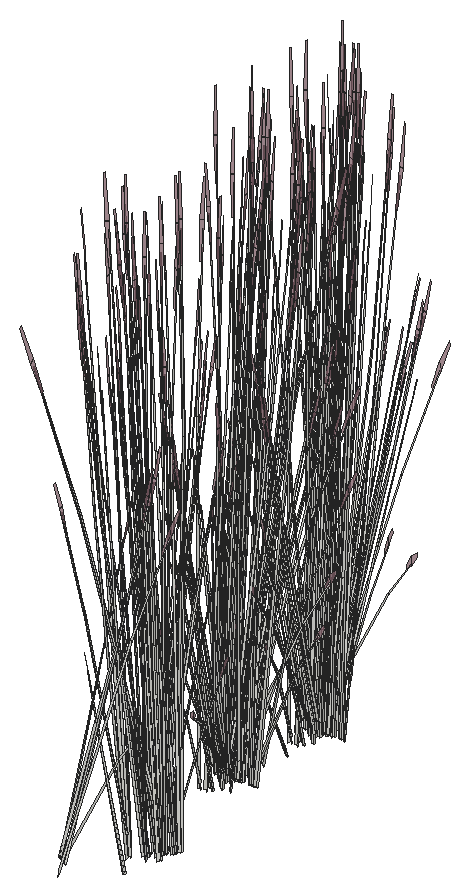
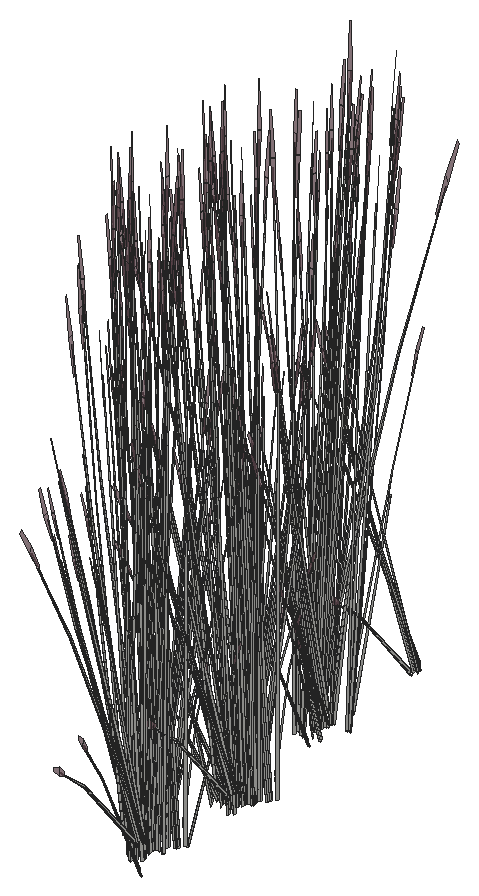
# SketchUp Ruby script. Lengths in inches.
U = 1.inch
M = Sketchup.active_model
def pt(a) = Geom::Point3d.new(a.map { |v| v * U })
def face(e, loops, mat)
  f = e.add_face(loops[0].map { |a| pt(a) })
  loops[1..].each { |l| e.add_face(l.map { |a| pt(a) }).erase! }
  f.material = f.back_material = mat if mat
  f
end
# faces: each face lists its corners as indices into pts; further lists are holes
def faces(e, pts, list, mat = nil) = list.each { |f| face(e, (f[0].is_a?(Array) ? f : [f]).map { |l| l.map { |i| pts[i] } }, mat) }
# xy, xz, yz: faces in a plane at the given z, y or x. An outline is a flat list of corners, or four numbers for a rectangle; further outlines are holes
def ring(l) = l.size == 4 ? [[l[0], l[1]], [l[2], l[1]], [l[2], l[3]], [l[0], l[3]]] : l.each_slice(2).to_a
def flat(e, list, mat, &to3) = list.each { |f| face(e, (f[0].is_a?(Array) ? f : [f]).map { |l| ring(l).map { |u, v| to3.(u, v) } }, mat) }
def xy(e, z, list, mat = nil) = flat(e, list, mat) { |x, y| [x, y, z] }
def xz(e, y, list, mat = nil) = flat(e, list, mat) { |x, z| [x, y, z] }
def yz(e, x, list, mat = nil) = flat(e, list, mat) { |y, z| [x, y, z] }
def lines(e, pts, list) = list.each { |a, b| e.add_line(pt(pts[a]), pt(pts[b])) }
# prism: a flat outline (further loops are holes) pulled along v
def prism(e, loops, v, mat = nil)
  f = face(e, loops, mat); d = Geom::Vector3d.new(v.map { |x| x * U })
  f.pushpull(f.normal.samedirection?(d) ? d.length : -d.length)
end
def box(e, o, s, mat = nil) = prism(e, [[o, [o[0] + s[0], o[1], o[2]], [o[0] + s[0], o[1] + s[1], o[2]], [o[0], o[1] + s[1], o[2]]]], [0, 0, s[2]], mat)
def at(x, y, z, deg = 0) = Geom::Transformation.translation(pt([x, y, z])) * Geom::Transformation.rotation(ORIGIN, Z_AXIS, deg.degrees)
def axes(o, x, y, z) = Geom::Transformation.new([*x, 0, *y, 0, *z, 0, *pt(o).to_a, 1])
def part(name) = M.definitions.add(name)
# library, detail: a bought-in or finely detailed component or shape, given as its bounding box
def library(name, o, s) = part(name).tap { |d| box(d.entities, o, s) }
def detail(e, o, s) = box(e.add_group.entities, o, s)
def put(e, d, t, mat = nil) = e.add_instance(d, t).tap { |i| i.material = mat if mat }
def group(e, t, mat = nil) = e.add_group.tap { |g| g.transformation = t; g.material = mat if mat }.entities
root = M.entities
M.materials.add("LightPink_Translucent").color = [144, 107, 117]
M.materials["LightPink_Translucent"].alpha = 0.75
c1 = part("blade")
p = [[2.15,0.21,22],[0,0.17,0],[0.09,0.45,0],[2.18,0.31,22],[2.29,0.31,22],[0.38,0.45,0],
  [2.48,0.24,33],[2.49,0.24,33],[2.48,0.22,33]]
faces(c1.entities,p,[[0,1,2,3],[4,5,2,3],[6,3,4,7],[8,0,3,6]])
c2 = part("seeds")
p = [[0.3,-0.1,1.38],[-0.01,-0.03,1.59],[-0.01,-0.03,0.03],[0.14,-0.07,-0.07],[0.29,-0.03,3],[0.15,0.01,3.11]]
faces(c2.entities,p,[[0,1,2,3],[1,0,4,5]],"LightPink_Translucent")
c3 = part("blade with seeds")
put(c3.entities,c1,at(0,0,0))
put(c3.entities,c2,axes([2.4,0.25,30.99],[1.5799,-0.05474,1.17369],[-0.12525,1.92788,0.29478],[-0.07173,-0.02425,1.56792]))
put(root,c3,axes([405.5625,393.34,-10.02],[-0.35341,0.31182,-0.03625],[-0.32382,-0.34152,-0.16435],[-0.0228,-0.09677,0.54209]))
put(root,c3,axes([403.33,388.5,-7.64],[0.50273,0.13626,-0.47583],[-0.17232,0.46717,-0.36857],[0.0461,0.18809,0.91046]))
put(root,c3,axes([403.61,387.54,-8.39],[-0.1169,-0.17452,1.59586],[0.54019,-0.14692,0.12904],[0.12209,0.27397,0.68222]))
put(root,c3,axes([406.02,397.03,-8.9],[0.44194,0.21918,1.40854],[-0.43295,0.47219,0.557],[-0.19393,-0.27986,1.18082]))
put(root,c3,axes([403.1,388.79,-7.78],[-0.15418,0.41799,-0.32977],[-0.44981,-0.12192,0.42575],[0.04124,0.16829,0.81462]))
put(root,c3,axes([405.09,394.07,-7.3],[0.07899,0.43781,0.32977],[-0.45153,0.11561,-0.42575],[-0.12128,-0.12546,0.81462]))
put(root,c3,axes([403.71,395.52,-10.12],[0,-0.54355,-0.46235],[0.57217,0,0],[0,-0.1238,1.46668]))
put(root,c3,axes([403.14,388.41,-7.36],[0.24409,0.44196,-0.66157],[-0.50245,0.2463,0.07984],[0.05708,0.21354,0.93586]))
put(root,c3,axes([405.26,395.74,-9.94],[0.24813,-0.48978,-0.41661],[0.51557,0.23571,0.2005],[0,-0.1129,1.33761]))
put(root,c3,axes([403.95,395.53,-10.11],[0.35699,-0.33913,-0.28847],[0.35699,0.33913,0.28847],[0,-0.10923,1.29413]))
put(root,c3,axes([402.78,389.53,-7.61],[0.06483,0.08753,1.62908],[0.52315,0.03439,-0.25764],[0.05261,0.19303,0.13065]))
put(root,c3,axes([405.2,396.15,-9.52],[-0.57594,-0.25935,-0.27094],[0.27732,-0.5474,-0.46562],[-0.0181,-0.1344,1.4872]))
put(root,c3,axes([404.06,395.77,-9.83],[-0.47569,0.45698,0.2864],[-0.47598,-0.45217,-0.33981],[-0.01661,-0.12977,1.53541]))
put(root,c3,axes([405.35,396.72,-9.73],[0.13555,-0.64407,-0.21817],[0.64269,0.11227,0.47743],[-0.1123,-0.08895,1.45677]))
put(root,c3,axes([403.95,396.02,-9.69],[0,0.54355,0.46235],[-0.57217,0,0],[0,-0.1238,1.46668]))
put(root,c3,axes([405.3,396.46,-9.94],[-0.30722,-0.45622,-0.41661],[0.46535,-0.32126,0.2005],[-0.09942,-0.05645,1.33761]))
put(root,c3,axes([405.37,395.82,-9.8],[0.22235,0.6078,0.42607],[-0.63531,0.21135,0.16719],[0.00776,-0.11168,1.47927]))
put(root,c3,axes([405.25,396.3,-9.47],[-0.24813,0.48978,0.41661],[-0.51557,-0.23571,-0.2005],[0,-0.1129,1.33761]))
put(root,c3,axes([406.33,396.36,-9.86],[-0.47569,-0.46784,-0.05709],[0.47598,-0.46812,0],[-0.01661,-0.01634,1.63492]))
put(root,c3,axes([405.42,396.41,-9.8],[0.64638,0.11452,0.42607],[-0.13155,0.64678,0.16719],[-0.09446,-0.06245,1.47927]))
put(root,c3,axes([405.07,397.45,-9.7],[0.54955,-0.14427,0.16428],[0.1357,0.53689,0.32672],[-0.04901,-0.07823,1.49371]))
put(root,c3,axes([405.9,397.32,-9.95],[-0.16686,-0.46861,0],[0.47648,-0.16411,0],[0,0,1.4375]))
put(root,c3,axes([405.58,396.875,-9.5625],[-0.09866,0.48509,0.13483],[-0.48202,-0.0842,-0.38503],[-0.08772,-0.04981,1.18024]))
put(root,c3,axes([406.71,397.48,-9.7],[0.14774,-0.54019,0.16428],[0.54062,0.15287,0.32672],[-0.09339,0.00263,1.49371]))
put(root,c3,axes([405.78,397.53,-9.95],[-0.51557,-0.24403,0],[0.24813,-0.50705,0],[0,0,1.51513]))
put(root,c3,axes([406.21,396.88,-9.7],[-0.49938,-0.43748,-0.23459],[0.42021,-0.49126,0.51337],[-0.13447,0.05118,1.56642]))
put(root,c3,axes([404.9,397.72,-9.69],[0.47863,0.27177,0.46235],[-0.28609,0.48733,0],[-0.10901,-0.0619,1.46668]))
put(root,c3,axes([406.45,396.52,-9.47],[0.55535,-0.03355,0.41661],[0.05022,0.55698,-0.2005],[-0.09942,0.05645,1.33761]))
put(root,c3,axes([405.96,396.79,-9.94],[-0.55535,0.03355,-0.41661],[-0.05022,-0.55698,0.2005],[-0.09942,0.05645,1.33761]))
put(root,c3,axes([406.57,398.08,-9.96],[-0.31576,-0.54657,-0.04789],[0.53494,-0.30375,0.48057],[-0.13182,0.05204,1.52373]))
put(root,c3,axes([406.46,396.76,-9.5625],[0.37783,0.32657,0.13483],[-0.31516,0.36844,-0.38503],[-0.08772,0.04981,1.18024]))
put(root,c3,axes([406.86,397.76,-9.69],[0.47863,-0.27177,0.46235],[0.28609,0.48733,0],[-0.10901,0.0619,1.46668]))
put(root,c3,axes([406.43,398.01,-10.11],[-0.47712,-0.13449,-0.28847],[0.12013,-0.47362,0.28847],[-0.09619,0.05462,1.29413]))
put(root,c3,axes([406.35,396.64,-9.52],[0.05959,0.62022,-0.27094],[-0.62068,0.0375,-0.46562],[-0.1093,0.08261,1.4872]))
put(root,c3,axes([406.57,396.4,-9.94],[-0.24813,0.48978,-0.41661],[-0.51557,-0.23571,0.2005],[0,0.1129,1.33761]))
put(root,c3,axes([405.97,397.11,-10.08],[-0.34446,0.40855,-0.58063],[-0.42791,-0.37046,-0.15239],[-0.13803,0.10191,1.28164]))
put(root,c3,axes([406.59,397.8,-9.83],[0.64025,0.17667,0.2864],[-0.16018,0.63149,-0.33981],[-0.10597,0.07904,1.53541]))
put(root,c3,axes([406.54,398.23,-10.12],[-0.47863,0.27177,-0.46235],[-0.28609,-0.48733,0],[-0.10901,0.0619,1.46668]))
put(root,c3,axes([404.38,397.5625,-7.3],[0.34603,-0.28618,0.32977],[0.32756,0.32677,-0.42575],[-0.04984,0.16603,0.81462]))
put(root,c3,axes([406.98,398.14,-9.79],[0.31974,0.54466,0],[-0.53494,0.30375,-0.48057],[-0.12184,0.06918,1.52448]))
put(root,c3,axes([406.7,395.99,-9.35],[-0.01397,-0.51177,1.31553],[0.63227,0.13266,0.557],[-0.14954,0.28003,1.24175]))
put(root,c3,axes([405.21,398.41,-7.6],[-0.37684,0.18473,0.05988],[-0.18445,-0.33686,0.47138],[0.03639,0.14849,0.71878]))
put(root,c3,axes([404.16,397.64,-6.97],[0.56206,0.02693,-0.12569],[-0.01536,0.50991,-0.69765],[-0.03904,0.19638,1.06006]))
put(root,c3,axes([405.35,398.375,-7.28],[-0.50393,-0.1421,0.49617],[0.17232,-0.46717,0.40911],[0.03028,0.18372,1.0267]))
put(root,c3,axes([404.42,399.08,-9.42],[-0.01324,-0.32319,1.06958],[0.33072,0.23052,0.78586],[-0.06504,0.15405,0.23558]))
put(root,c3,axes([405.29,398.31,-10.61],[0.08277,-0.02958,1.6421],[0.49786,0.16279,-0.25086],[0.01456,0.18348,0.2797]))
put(root,c3,axes([404.55,397.83,-7.34],[0.3661,0.36521,-0.52818],[-0.38674,0.31985,-0.40911],[-0.0557,0.18556,1.01061]))
put(root,c3,axes([404.15,398.38,-9.37],[0.46459,-0.09625,0.0606],[0.10681,0.38778,-0.80367],[-0.02945,0.1963,0.72038]))
put(root,c3,axes([405.4,398.47,-7.78],[-0.15418,0.41799,-0.32977],[-0.44981,-0.12192,0.42575],[0.04124,0.16829,0.81462]))
put(root,c3,axes([404.43,397.67,-7.03],[-0.01331,0.50278,-0.73435],[-0.56035,-0.03377,0.08862],[-0.05914,0.213,1.03881]))
put(root,c3,axes([402.97,398.99,-7.62],[0.05802,-0.03282,1.65179],[0.47954,0.21828,-0.15608],[-0.01127,0.18175,0.29231]))
put(root,c3,axes([404.96,397.31,-8.39],[-0.01252,-0.20862,1.59586],[0.54251,0.1384,0.12904],[-0.03356,0.2973,0.68222]))
put(root,c3,axes([403.35,406.68,-9.59],[-0.14537,0.11002,1.33163],[-0.43536,-0.19256,-0.28638],[0.0807,-0.23948,0.56934]))
put(root,c3,axes([403.7,407.5,-7.36],[0.01331,-0.50278,-0.66157],[0.56035,0.03377,0.07984],[0.05914,-0.213,0.93586]))
put(root,c3,axes([404.48,406.71,-7.61],[-0.00494,-0.10818,1.62908],[-0.41695,-0.31265,-0.25764],[0.06446,-0.18952,0.13065]))
put(root,c3,axes([403.07,407.24,-8.39],[-0.09522,0.18683,1.59586],[-0.39947,-0.38663,0.12904],[0.18021,-0.24097,0.68222]))
put(root,c3,axes([404.37,406.32,-7.62],[-0.05194,0.04152,1.65179],[-0.50886,-0.14007,-0.15608],[-0.01842,-0.18118,0.29231]))
put(root,c3,axes([402.8125,405.81,-9.42],[0.06561,0.31695,1.06958],[-0.36394,-0.17555,0.78586],[0.03916,-0.16229,0.23558]))
put(root,c3,axes([403.59,407.33,-7.64],[-0.3661,-0.36521,-0.47583],[0.38674,-0.31985,-0.36857],[0.0557,-0.18556,0.91046]))
put(root,c3,axes([404.25,398.375,-8.87],[0.01124,-0.2806,1.43727],[0.50537,0.14821,0.19862],[-0.04379,0.29905,0.67868]))
put(root,c3,axes([402.79,406.79,-7.59],[0.50393,0.1421,0.447],[-0.17232,0.46717,0.36857],[-0.03028,-0.18372,0.92496]))
put(root,c3,axes([403.97,407.52,-7.3125],[-0.56206,-0.02693,-0.11324],[0.01536,-0.50991,-0.62851],[0.03904,-0.19638,0.95501]))
put(root,c3,axes([403.93,407.19,-7.78],[0.34603,-0.28618,-0.32977],[0.32756,0.32677,0.42575],[0.04984,-0.16603,0.81462]))
put(root,c3,axes([402.92,406.75,-7.6],[0.37684,-0.18473,0.05988],[0.18445,0.33686,0.47138],[-0.03639,-0.14849,0.71878]))
put(root,c3,axes([403.93,407.31,-7.59],[0.36417,0.37086,0.447],[-0.38674,0.31985,0.36857],[0.06718,-0.174,0.92496]))
put(root,c3,axes([404.0625,407.34,-7.6],[0.42027,0.02533,0.05988],[-0.01152,0.38243,0.47138],[0.04398,-0.14649,0.71878]))
put(root,c3,axes([403.75,407.6,-7.3],[-0.34603,0.28618,0.32977],[-0.32756,-0.32677,-0.42575],[0.04984,-0.16603,0.81462]))
put(root,c3,axes([401.47,407.12,-9.79],[-0.31974,-0.54466,0],[0.53494,-0.30375,-0.48057],[0.12184,-0.06918,1.52448]))
put(root,c3,axes([401.91,407.04,-10.12],[0.47863,-0.27177,-0.46235],[0.28609,0.48733,0],[0.10901,-0.0619,1.46668]))
put(root,c3,axes([402.47,408.15,-10.08],[0.34446,-0.40855,-0.58063],[0.42791,0.37046,-0.15239],[0.13803,-0.10191,1.28164]))
put(root,c3,axes([402.1,408.625,-9.52],[-0.05959,-0.62022,-0.27094],[0.62068,-0.0375,-0.46562],[0.1093,-0.08261,1.4872]))
put(root,c3,axes([404.35,408.48,-7.3],[-0.44516,0.07768,0.32977],[-0.11755,-0.44407,-0.42575],[0.12757,-0.11927,0.81462]))
put(root,c3,axes([402.02,407.25,-10.11],[0.47712,0.13449,-0.28847],[-0.12013,0.47362,0.28847],[0.09619,-0.05462,1.29413]))
put(root,c3,axes([402.18,409.11,-9.73],[0.57623,0.26344,0.22409],[-0.27732,0.5474,0.46562],[0,-0.12618,1.49497]))
put(root,c3,axes([402,408.74,-9.47],[-0.55535,0.03355,0.41661],[-0.05022,-0.55698,-0.2005],[0.09942,-0.05645,1.33761]))
put(root,c3,axes([402.78,409,-9.95],[0,-0.62892,0],[0.63949,0,0],[0,0,1.6711]))
put(root,c3,axes([403.55,407.54,-9.69],[-0.47863,-0.27177,0.46235],[0.28609,-0.48733,0],[0.10901,0.0619,1.46668]))
put(root,c3,axes([402.47,408.6,-9.8],[-0.42403,0.49328,0.42607],[-0.50377,-0.43543,0.16719],[0.10223,-0.04923,1.47927]))
put(root,c3,axes([401.74,407.79,-9.7],[-0.14774,0.54019,0.16428],[-0.54062,-0.15287,0.32672],[0.09339,-0.00263,1.49371]))
put(root,c3,axes([402.87,408.39,-9.5625],[0.09866,-0.48509,0.13483],[0.48202,0.0842,-0.38503],[0.08772,0.04981,1.18024]))
put(root,c3,axes([402.66,408.52,-9.47],[-0.30722,-0.45622,0.41661],[0.46535,-0.32126,-0.2005],[0.09942,0.05645,1.33761]))
put(root,c3,axes([402.82,408.55,-9.52],[0.51635,-0.36087,-0.27094],[0.34336,0.5099,-0.46562],[0.1274,0.05178,1.4872]))
put(root,c3,axes([403.21,409.14,-9.95],[0.57217,0,0],[0,0.56272,0],[0,0,1.66132]))
put(root,c3,axes([403.37,407.82,-9.7],[-0.54955,0.14427,0.16428],[-0.1357,-0.53689,0.32672],[0.04901,0.07823,1.49371]))
put(root,c3,axes([403.99,407.79,-10.11],[0.12013,0.47362,-0.28847],[-0.47712,0.13449,0.28847],[0.09619,0.05462,1.29413]))
put(root,c3,axes([403.03,408.85,-9.78],[-0.64638,-0.11452,0.45814],[0.13155,-0.64678,0.17978],[0.09446,0.06245,1.59061]))
put(root,c3,axes([403.13,410.38,-9.97],[0.53691,-0.18442,-0.17877],[0.18866,0.53125,0.00007],[0.05927,-0.02038,1.61933]))
put(root,c3,axes([403.2,409.38,-9.9375],[0.35699,0.35109,0],[-0.35699,0.35109,0],[0,0,1.57621]))
put(root,c3,axes([404.16,409.23,-9.7],[-0.40181,-0.39593,0.16428],[0.40492,-0.38402,0.32672],[-0.04438,0.08086,1.49371]))
put(root,c3,axes([403.19,408.97,-9.47],[0.24813,-0.48978,0.41661],[0.51557,0.23571,-0.2005],[0,0.1129,1.33761]))
put(root,c3,axes([403.1,409.25,-9.87],[0,0.62861,-0.05249],[-0.63949,0,0],[0,0.01975,1.67027]))
put(root,c3,axes([403.14,408.8,-9.94],[0.30722,0.45622,-0.41661],[-0.46535,0.32126,0.2005],[0.09942,0.05645,1.33761]))
put(root,c3,axes([404.49,409.24,-9.69],[0,-0.54355,0.46235],[0.57217,0,0],[0,0.1238,1.46668]))
put(root,c3,axes([403.41,409.08,-9.5625],[0.47648,-0.15851,0.13483],[0.16686,0.45265,-0.38503],[0,0.09962,1.18024]))
put(root,c3,axes([402.98,410.67,-9.95],[0.51557,0.24403,0],[-0.24813,0.50705,0],[0,0,1.62917]))
put(root,c3,axes([402.79,410.46,-9.87],[0.22235,0.62444,-0.05599],[-0.63531,0.21881,0],[0.00776,0.02181,1.60327]))
put(root,c3,axes([404.88,409.33,-9.79],[0.63949,0,0],[0,0.60749,-0.48057],[0,0.13836,1.52448]))
put(root,c3,axes([404.63,409.64,-9.95],[-0.63917,-0.00435,-0.04634],[0,-0.60749,0.46507],[-0.02009,0.13829,1.47457]))
put(root,c3,axes([403.24,409.12,-9.52],[0.57594,0.25935,-0.27094],[-0.27732,0.5474,-0.46562],[0.0181,0.1344,1.4872]))
put(root,c3,axes([404.3,416.28,-9.59],[-0.14537,0.11002,1.33163],[-0.43536,-0.19256,-0.28638],[0.0807,-0.23948,0.56934]))
put(root,c3,axes([404.49,409.73,-10.11],[-0.35699,0.33913,-0.28847],[-0.35699,-0.33913,0.28847],[0,0.10923,1.29413]))
put(root,c3,axes([403.21,415.68,-10.61],[-0.08578,0.01958,1.6421],[-0.47437,-0.22044,-0.25086],[0.00796,-0.18387,0.2797]))
put(root,c3,axes([404.65,417.1,-7.36],[0.01331,-0.50278,-0.66157],[0.56035,0.03377,0.07984],[0.05914,-0.213,0.93586]))
put(root,c3,axes([403.68,416.29,-7.78],[0.15418,-0.41799,-0.32977],[0.44981,0.12192,0.42575],[-0.04124,-0.16829,0.81462]))
put(root,c3,axes([405.32,415.92,-7.62],[-0.05194,0.04152,1.65179],[-0.50886,-0.14007,-0.15608],[-0.01842,-0.18118,0.29231]))
put(root,c3,axes([403.04,411.09,-7.3],[-0.07899,-0.43781,0.32977],[0.45153,-0.11561,-0.42575],[0.12128,0.12546,0.81462]))
put(root,c3,axes([404.74,409.75,-10.12],[0,0.54355,-0.46235],[-0.57217,0,0],[0,0.1238,1.46668]))
put(root,c3,axes([403.35,408.57,-7.83],[-0.44191,-0.28242,1.28769],[0.46662,-0.43971,0.5556],[0.14258,0.26499,1.24467]))
put(root,c3,axes([403.76,415.41,-9.42],[0.06561,0.31695,1.06958],[-0.36394,-0.17555,0.78586],[0.03916,-0.16229,0.23558]))
put(root,c3,axes([404.54,416.93,-7.64],[-0.3661,-0.36521,-0.47583],[0.38674,-0.31985,-0.36857],[0.0557,-0.18556,0.91046]))
put(root,c3,axes([404.01,410.87,-9.42],[-0.28795,-0.15629,1.06958],[0.37181,-0.1588,0.78586],[0.10029,0.13452,0.23558]))
put(root,c3,axes([403.74,416.39,-7.59],[0.50393,0.1421,0.447],[-0.17232,0.46717,0.36857],[-0.03028,-0.18372,0.92496]))
put(root,c3,axes([404.92,417.12,-7.3125],[-0.56206,-0.02693,-0.11324],[0.01536,-0.50991,-0.62851],[0.03904,-0.19638,0.95501]))
put(root,c3,axes([402.6,411.7,-7.62],[0.00151,-0.06581,1.65179],[0.43826,-0.29033,-0.15608],[0.15223,0.10363,0.29231]))
put(root,c3,axes([403.87,416.35,-7.6],[0.37684,-0.18473,0.05988],[0.18445,0.33686,0.47138],[-0.03639,-0.14849,0.71878]))
put(root,c3,axes([403.47,409.67,-10.05],[0.18752,0.49766,-0.6445],[-0.54017,0.17923,-0.16915],[0.02073,0.16852,1.42262]))
put(root,c3,axes([401.96,411.16,-7.3],[0.15418,-0.41799,0.32977],[0.44981,0.12192,-0.42575],[0.04124,0.16829,0.81462]))
put(root,c3,axes([404.06,411.58,-9.52],[-0.32795,-0.01705,0.97832],[0.21658,-0.36206,0.54015],[0.12956,0.12863,0.76741]))
put(root,c3,axes([403.11,411.49,-7.6],[-0.23243,0.34529,0.05988],[-0.331,-0.20103,0.47138],[0.10701,0.1107,0.71878]))
put(root,c3,axes([402.57,412.65,-6.74],[0.35341,-0.31182,-0.06041],[0.32382,0.34152,-0.27392],[0.0228,0.09677,0.90349]))
put(root,c3,axes([403.21,411.39,-7.59],[-0.50866,0.12474,0.447],[-0.08828,-0.48932,0.36857],[0.11963,0.14421,0.92496]))
put(root,c3,axes([402.99,410.71,-9.59],[0.00902,-0.18018,1.33163],[0.43127,-0.20126,-0.28638],[0.13313,0.21566,0.56934]))
put(root,c3,axes([401.8125,411.34,-7.3125],[0.50045,-0.25306,-0.11324],[0.24593,0.44915,-0.62851],[0.06603,0.18927,0.95501]))
put(root,c3,axes([404.7,417.2,-7.3],[-0.34603,0.28618,0.32977],[-0.32756,-0.32677,-0.42575],[0.04984,-0.16603,0.81462]))
put(root,c3,axes([402.42,416.72,-9.79],[-0.31974,-0.54466,0],[0.53494,-0.30375,-0.48057],[0.12184,-0.06918,1.52448]))
put(root,c3,axes([402.24,411.31,-7.64],[0.50273,0.13626,-0.47583],[-0.17232,0.46717,-0.36857],[0.0461,0.18809,0.91046]))
put(root,c3,axes([402.53,410.35,-8.39],[-0.1169,-0.17452,1.59586],[0.54019,-0.14692,0.12904],[0.12209,0.27397,0.68222]))
put(root,c3,axes([402.86,416.64,-10.12],[0.47863,-0.27177,-0.46235],[0.28609,0.48733,0],[0.10901,-0.0619,1.46668]))
put(root,c3,axes([402.82,418.47,-9.94],[0.24813,-0.48978,-0.41661],[0.51557,0.23571,0.2005],[0,-0.1129,1.33761]))
put(root,c3,axes([402.06,411.23,-7.36],[0.24409,0.44196,-0.66157],[-0.50245,0.2463,0.07984],[0.05708,0.21354,0.93586]))
put(root,c3,axes([403.05,418.23,-9.52],[-0.05959,-0.62022,-0.27094],[0.62068,-0.0375,-0.46562],[0.1093,-0.08261,1.4872]))
put(root,c3,axes([401.69,412.34,-7.61],[0.06483,0.08753,1.62908],[0.52315,0.03439,-0.25764],[0.05261,0.19303,0.13065]))
put(root,c3,axes([402.97,416.85,-10.11],[0.47712,0.13449,-0.28847],[-0.12013,0.47362,0.28847],[0.09619,-0.05462,1.29413]))
put(root,c3,axes([403.13,418.71,-9.73],[0.57623,0.26344,0.22409],[-0.27732,0.5474,0.46562],[0,-0.12618,1.49497]))
put(root,c3,axes([402.95,418.35,-9.47],[-0.55535,0.03355,0.41661],[-0.05022,-0.55698,-0.2005],[0.09942,-0.05645,1.33761]))
put(root,c3,axes([402.93,418.55,-9.8],[0.22235,0.6078,0.42607],[-0.63531,0.21135,0.16719],[0.00776,-0.11168,1.47927]))
put(root,c3,axes([403.73,418.6,-9.95],[0,-0.62892,0],[0.63949,0,0],[0,0,1.6711]))
put(root,c3,axes([404.5,417.14,-9.69],[-0.47863,-0.27177,0.46235],[0.28609,-0.48733,0],[0.10901,0.0619,1.46668]))
put(root,c3,axes([403.42,418.2,-9.8],[-0.42403,0.49328,0.42607],[-0.50377,-0.43543,0.16719],[0.10223,-0.04923,1.47927]))
put(root,c3,axes([403.89,419.08,-9.86],[-0.47569,-0.46784,-0.05709],[0.47598,-0.46812,0],[-0.01661,-0.01634,1.63492]))
put(root,c3,axes([402.6875,417.39,-9.7],[-0.14774,0.54019,0.16428],[-0.54062,-0.15287,0.32672],[0.09339,-0.00263,1.49371]))
put(root,c3,axes([403.82,417.99,-9.5625],[0.09866,-0.48509,0.13483],[0.48202,0.0842,-0.38503],[0.08772,0.04981,1.18024]))
put(root,c3,axes([403.61,418.12,-9.47],[-0.30722,-0.45622,0.41661],[0.46535,-0.32126,-0.2005],[0.09942,0.05645,1.33761]))
put(root,c3,axes([404.16,418.74,-9.95],[0.57217,0,0],[0,0.56272,0],[0,0,1.66132]))
put(root,c3,axes([404.32,417.42,-9.7],[-0.54955,0.14427,0.16428],[-0.1357,-0.53689,0.32672],[0.04901,0.07823,1.49371]))
put(root,c3,axes([403.98,418.45,-9.78],[-0.64638,-0.11452,0.45814],[0.13155,-0.64678,0.17978],[0.09446,0.06245,1.59061]))
put(root,c3,axes([403.46,420.05,-9.95],[-0.16686,-0.46861,0],[0.47648,-0.16411,0],[0,0,1.4375]))
put(root,c3,axes([404.08,419.98,-9.97],[0.53691,-0.18442,-0.17877],[0.18866,0.53125,0.00007],[0.05927,-0.02038,1.61933]))
put(root,c3,axes([404.27,420.2,-9.7],[0.14774,-0.54019,0.16428],[0.54062,0.15287,0.32672],[-0.09339,0.00263,1.49371]))
put(root,c3,axes([404.15,418.98,-9.9375],[0.35699,0.35109,0],[-0.35699,0.35109,0],[0,0,1.57621]))
put(root,c3,axes([405.11,418.83,-9.7],[-0.40181,-0.39593,0.16428],[0.40492,-0.38402,0.32672],[-0.04438,0.08086,1.49371]))
put(root,c3,axes([404.14,418.57,-9.47],[0.24813,-0.48978,0.41661],[0.51557,0.23571,-0.2005],[0,0.1129,1.33761]))
put(root,c3,axes([404.05,418.85,-9.87],[0,0.62861,-0.05249],[-0.63949,0,0],[0,0.01975,1.67027]))
put(root,c3,axes([405.45,418.84,-9.69],[0,-0.54355,0.46235],[0.57217,0,0],[0,0.1238,1.46668]))
put(root,c3,axes([404.01,419.25,-9.47],[0.55535,-0.03355,0.41661],[0.05022,0.55698,-0.2005],[-0.09942,0.05645,1.33761]))
put(root,c3,axes([404.36,418.68,-9.5625],[0.47648,-0.15851,0.13483],[0.16686,0.45265,-0.38503],[0,0.09962,1.18024]))
put(root,c3,axes([403.93,420.27,-9.95],[0.51557,0.24403,0],[-0.24813,0.50705,0],[0,0,1.62917]))
put(root,c3,axes([404.02,419.49,-9.5625],[0.37783,0.32657,0.13483],[-0.31516,0.36844,-0.38503],[-0.08772,0.04981,1.18024]))
put(root,c3,axes([404.42,420.49,-9.69],[0.47863,-0.27177,0.46235],[0.28609,0.48733,0],[-0.10901,0.0619,1.46668]))
put(root,c3,axes([403.74,420.07,-9.87],[0.22235,0.62444,-0.05599],[-0.63531,0.21881,0],[0.00776,0.02181,1.60327]))
put(root,c3,axes([405.58,419.25,-9.95],[-0.63917,-0.00435,-0.04634],[0,-0.60749,0.46507],[-0.02009,0.13829,1.47457]))
put(root,c3,axes([404.2,418.72,-9.52],[0.57594,0.25935,-0.27094],[-0.27732,0.5474,-0.46562],[0.0181,0.1344,1.4872]))
put(root,c3,axes([405.45,419.33,-10.11],[-0.35699,0.33913,-0.28847],[-0.35699,-0.33913,0.28847],[0,0.10923,1.29413]))
put(root,c3,axes([404.13,419.125,-9.94],[-0.24813,0.48978,-0.41661],[-0.51557,-0.23571,0.2005],[0,0.1129,1.33761]))
put(root,c3,axes([403.99,420.69,-7.3],[-0.07899,-0.43781,0.32977],[0.45153,-0.11561,-0.42575],[0.12128,0.12546,0.81462]))
put(root,c3,axes([404.15,420.53,-9.83],[0.64025,0.17667,0.2864],[-0.16018,0.63149,-0.33981],[-0.10597,0.07904,1.53541]))
put(root,c3,axes([405.69,419.35,-10.12],[0,0.54355,-0.46235],[-0.57217,0,0],[0,0.1238,1.46668]))
put(root,c3,axes([404.43,419.27,-10.05],[0.18752,0.49766,-0.6445],[-0.54017,0.17923,-0.16915],[0.02073,0.16852,1.42262]))
put(root,c3,axes([402.91,420.76,-7.3],[0.15418,-0.41799,0.32977],[0.44981,0.12192,-0.42575],[0.04124,0.16829,0.81462]))
put(root,c3,axes([404.07,421.09,-7.6],[-0.23243,0.34529,0.05988],[-0.331,-0.20103,0.47138],[0.10701,0.1107,0.71878]))
put(root,c3,axes([403.52,422.25,-6.74],[0.35341,-0.31182,-0.06041],[0.32382,0.34152,-0.27392],[0.0228,0.09677,0.90349]))
put(root,c3,axes([404.16,420.99,-7.59],[-0.50866,0.12474,0.447],[-0.08828,-0.48932,0.36857],[0.11963,0.14421,0.92496]))
put(root,c3,axes([402.77,421.14,-7.6],[-0.37684,0.18473,0.05988],[-0.18445,-0.33686,0.47138],[0.03639,0.14849,0.71878]))
put(root,c3,axes([402.76,420.9375,-7.3125],[0.50045,-0.25306,-0.11324],[0.24593,0.44915,-0.62851],[0.06603,0.18927,0.95501]))
put(root,c3,axes([402.85,421.04,-10.61],[0.08277,-0.02958,1.6421],[0.49786,0.16279,-0.25086],[0.01456,0.18348,0.2797]))
put(root,c3,axes([403.19,420.92,-7.64],[0.50273,0.13626,-0.47583],[-0.17232,0.46717,-0.36857],[0.0461,0.18809,0.91046]))
put(root,c3,axes([403.48,419.95,-8.39],[-0.1169,-0.17452,1.59586],[0.54019,-0.14692,0.12904],[0.12209,0.27397,0.68222]))
put(root,c3,axes([402.96,421.2,-7.78],[-0.15418,0.41799,-0.32977],[-0.44981,-0.12192,0.42575],[0.04124,0.16829,0.81462]))
put(root,c3,axes([403.01,420.83,-7.36],[0.24409,0.44196,-0.66157],[-0.50245,0.2463,0.07984],[0.05708,0.21354,0.93586]))
put(root,c3,axes([402.65,421.94,-7.61],[0.06483,0.08753,1.62908],[0.52315,0.03439,-0.25764],[0.05261,0.19303,0.13065]))
